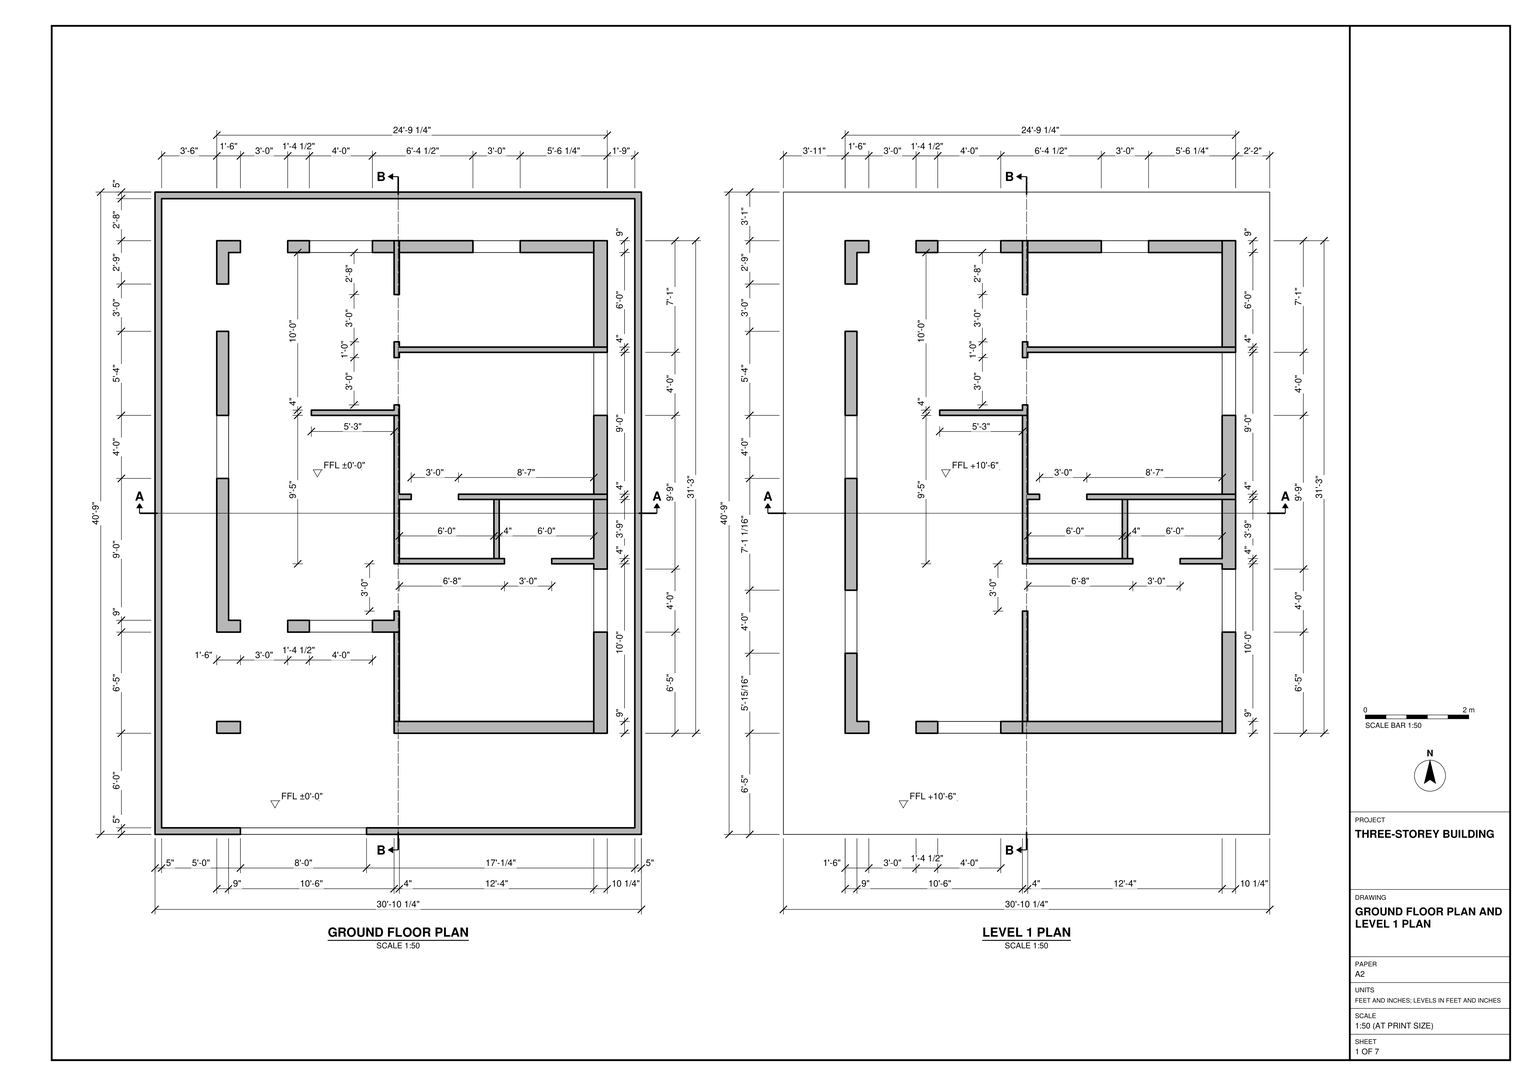
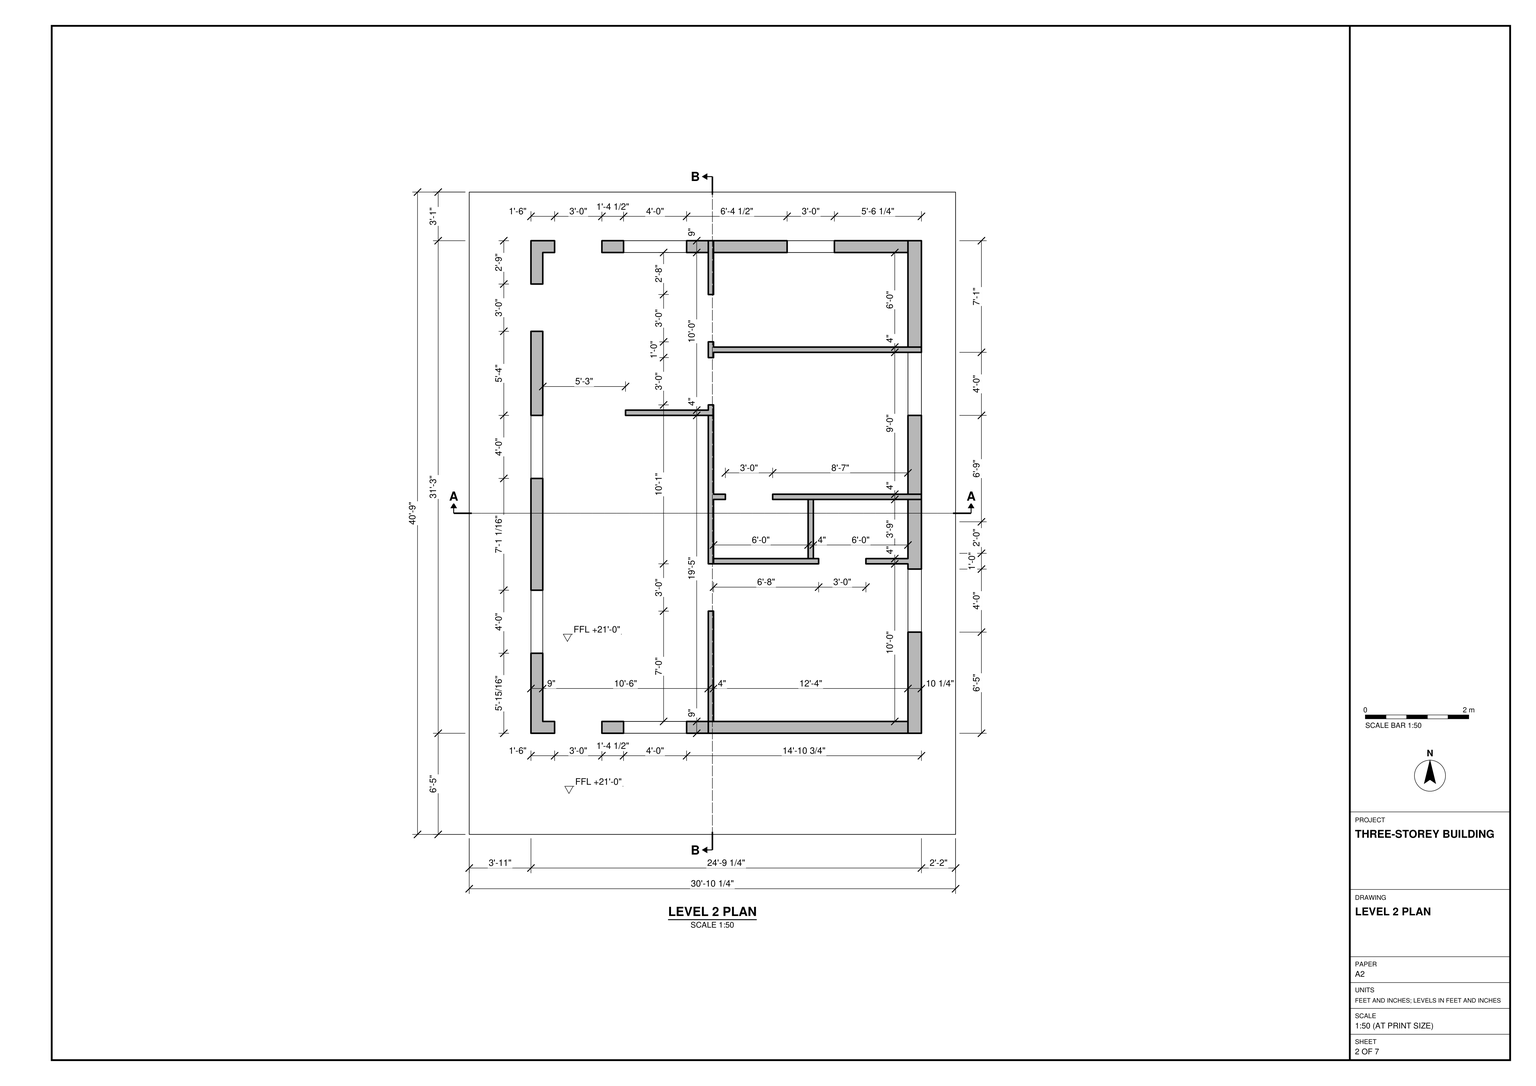
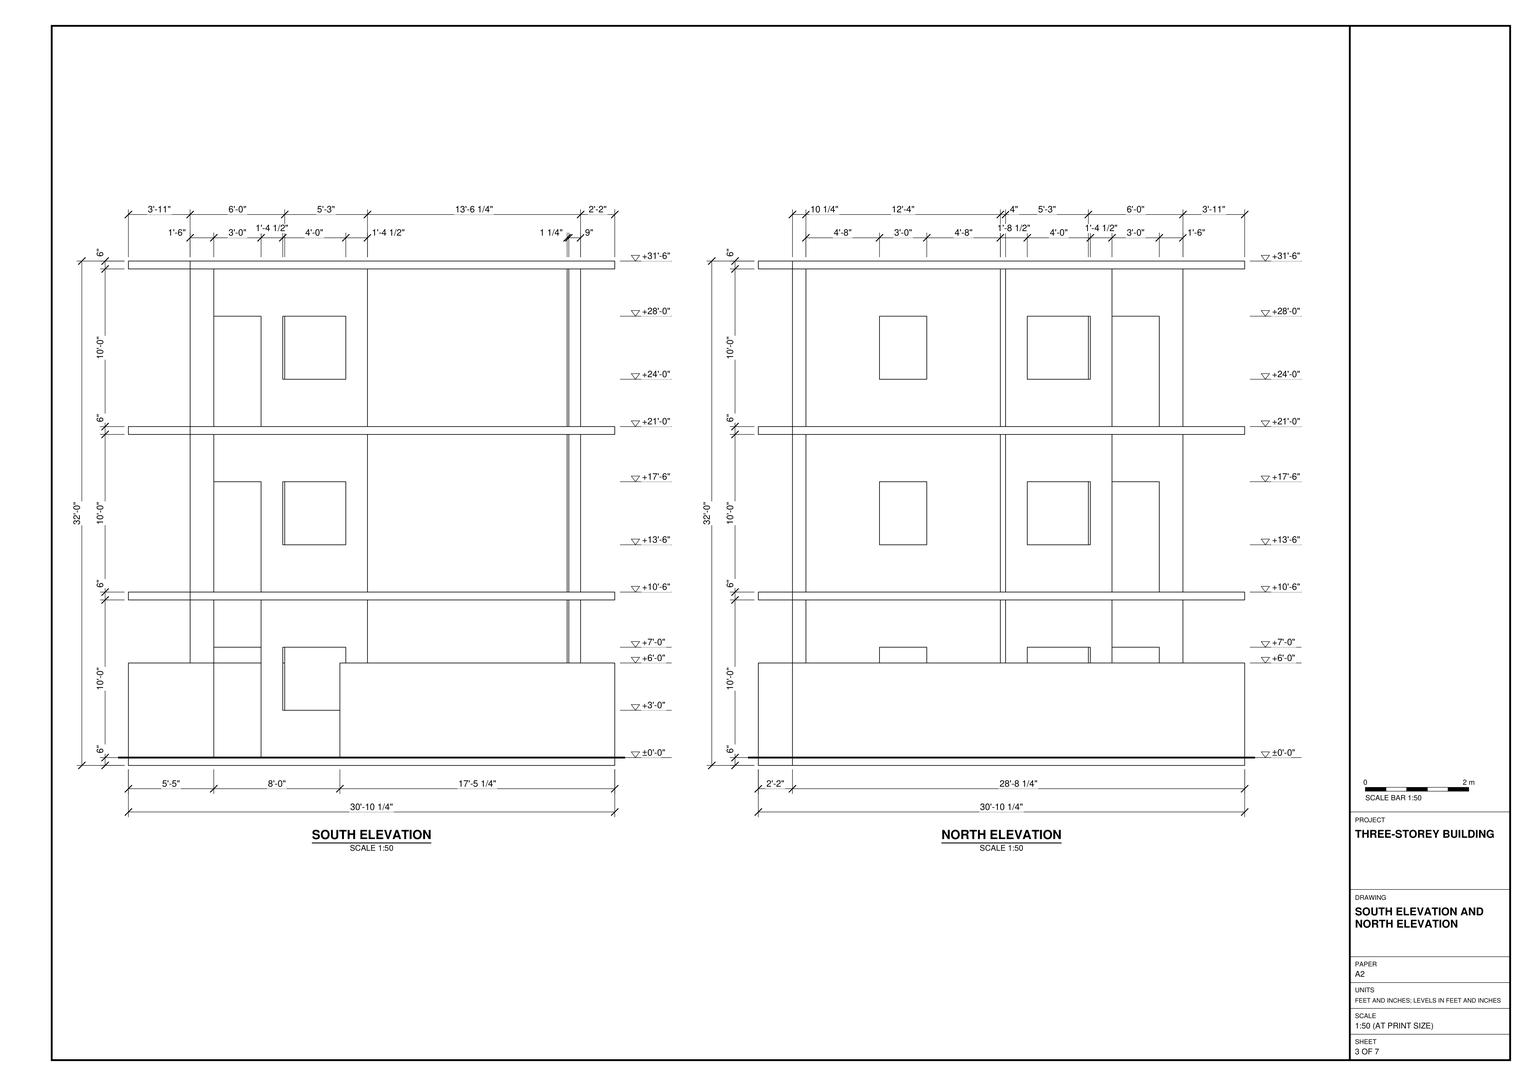
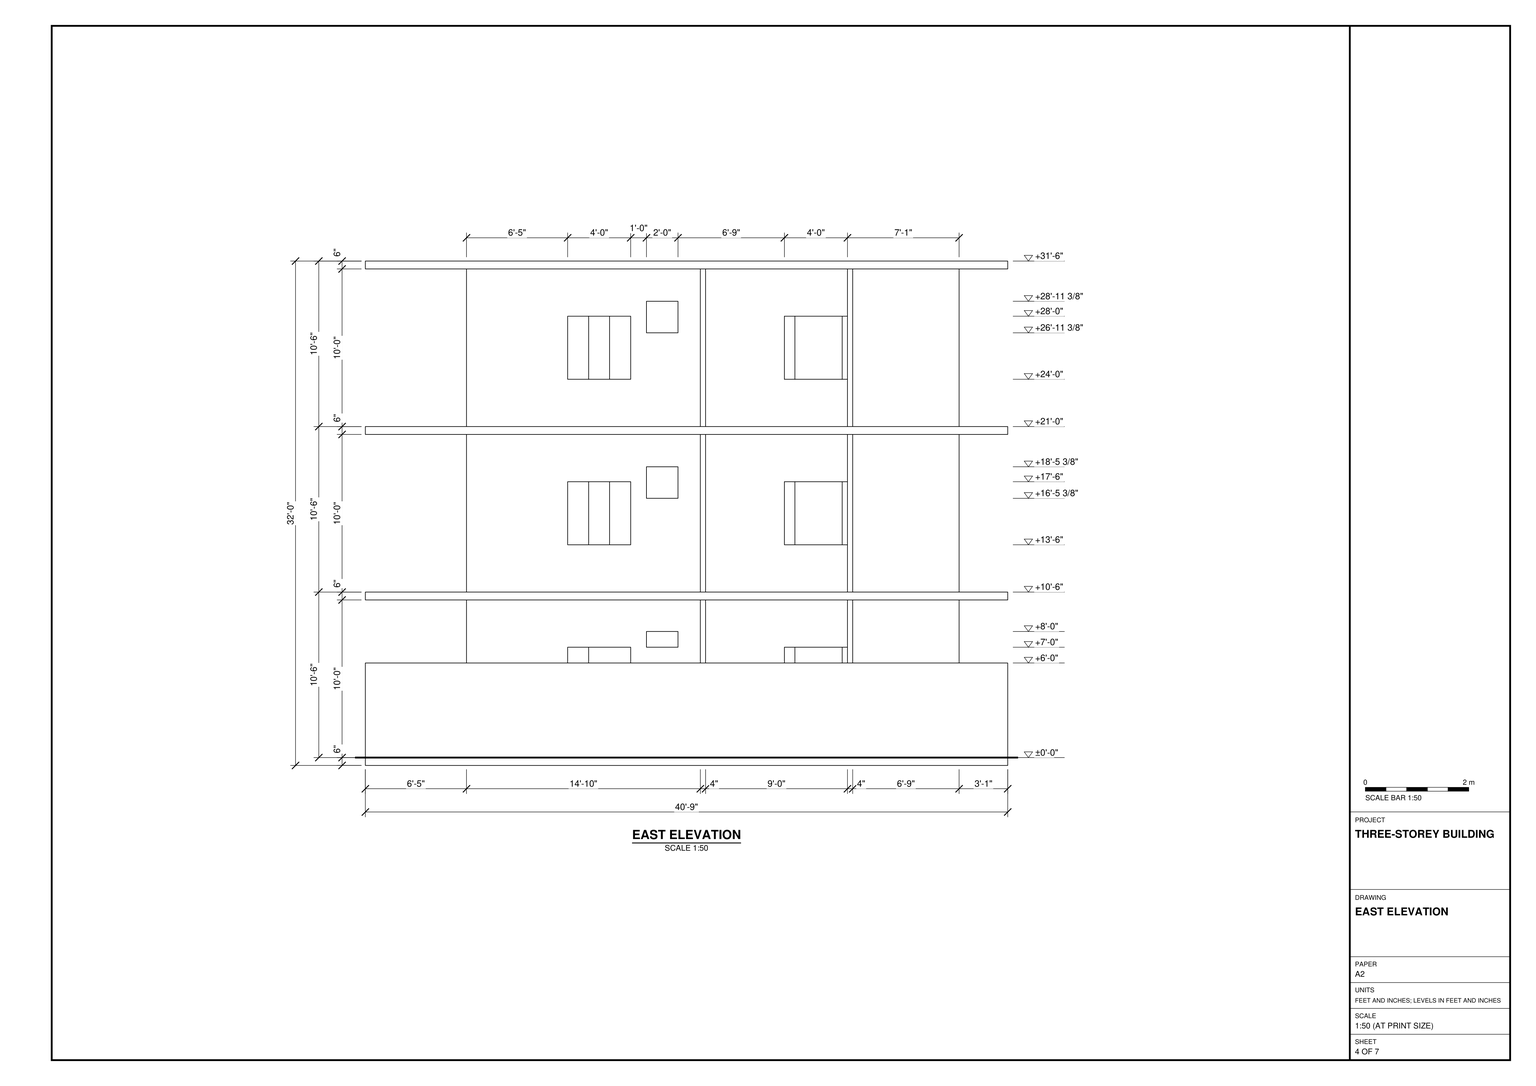
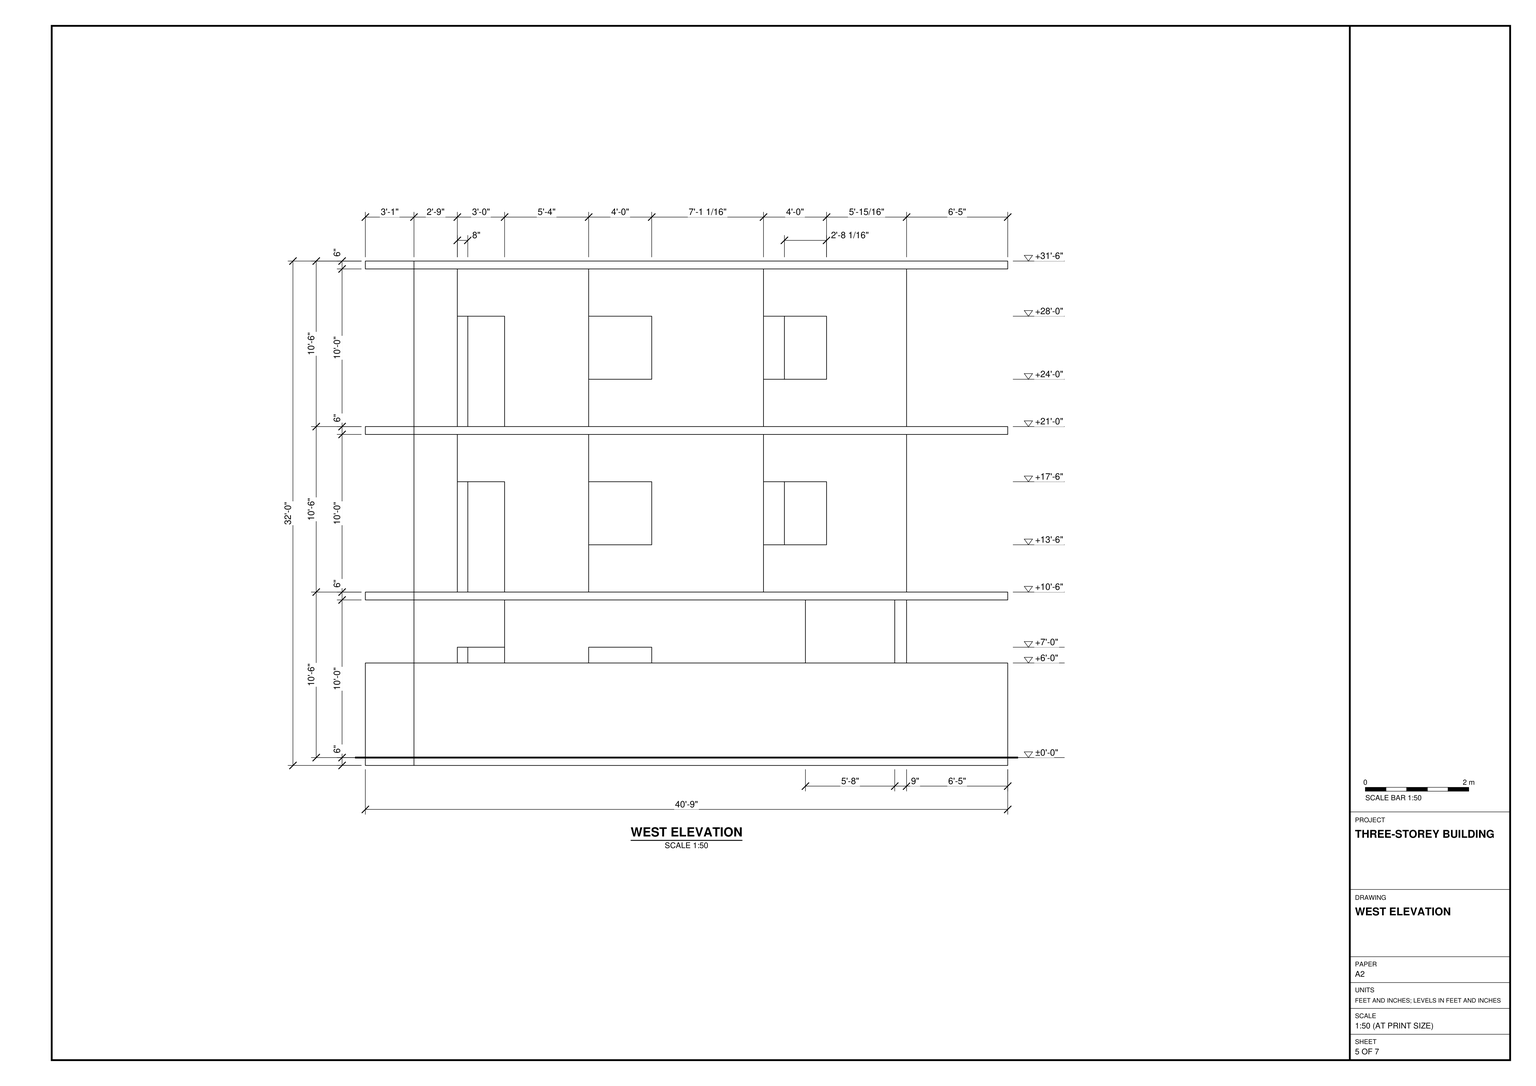
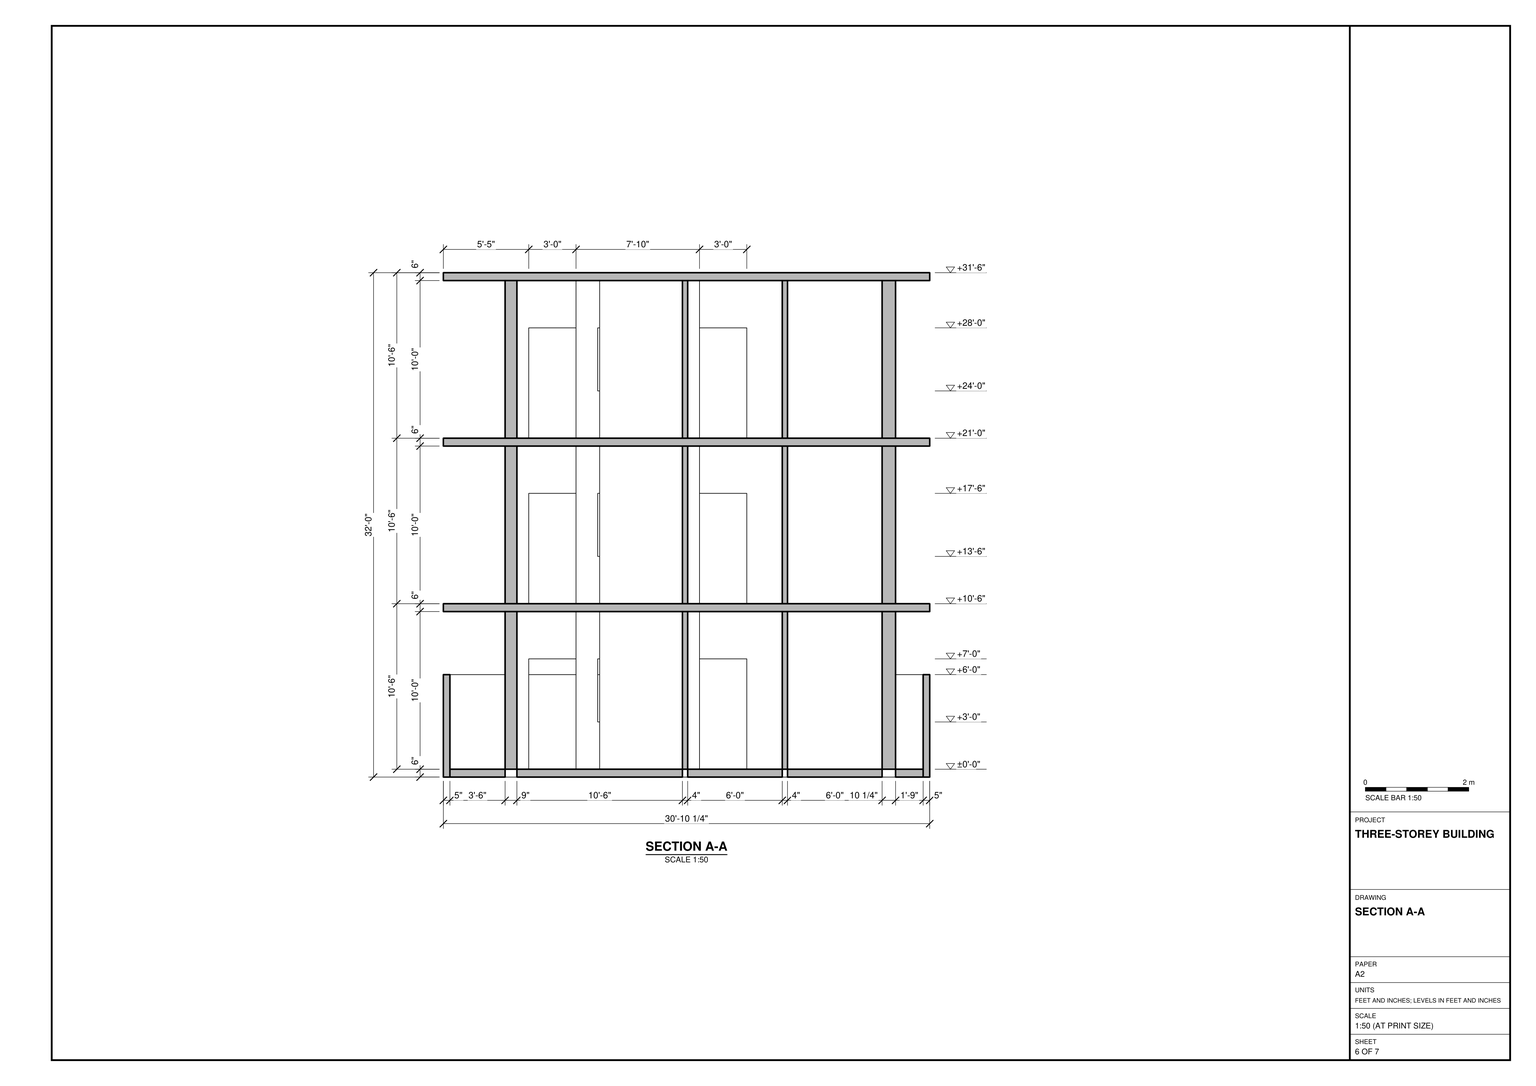
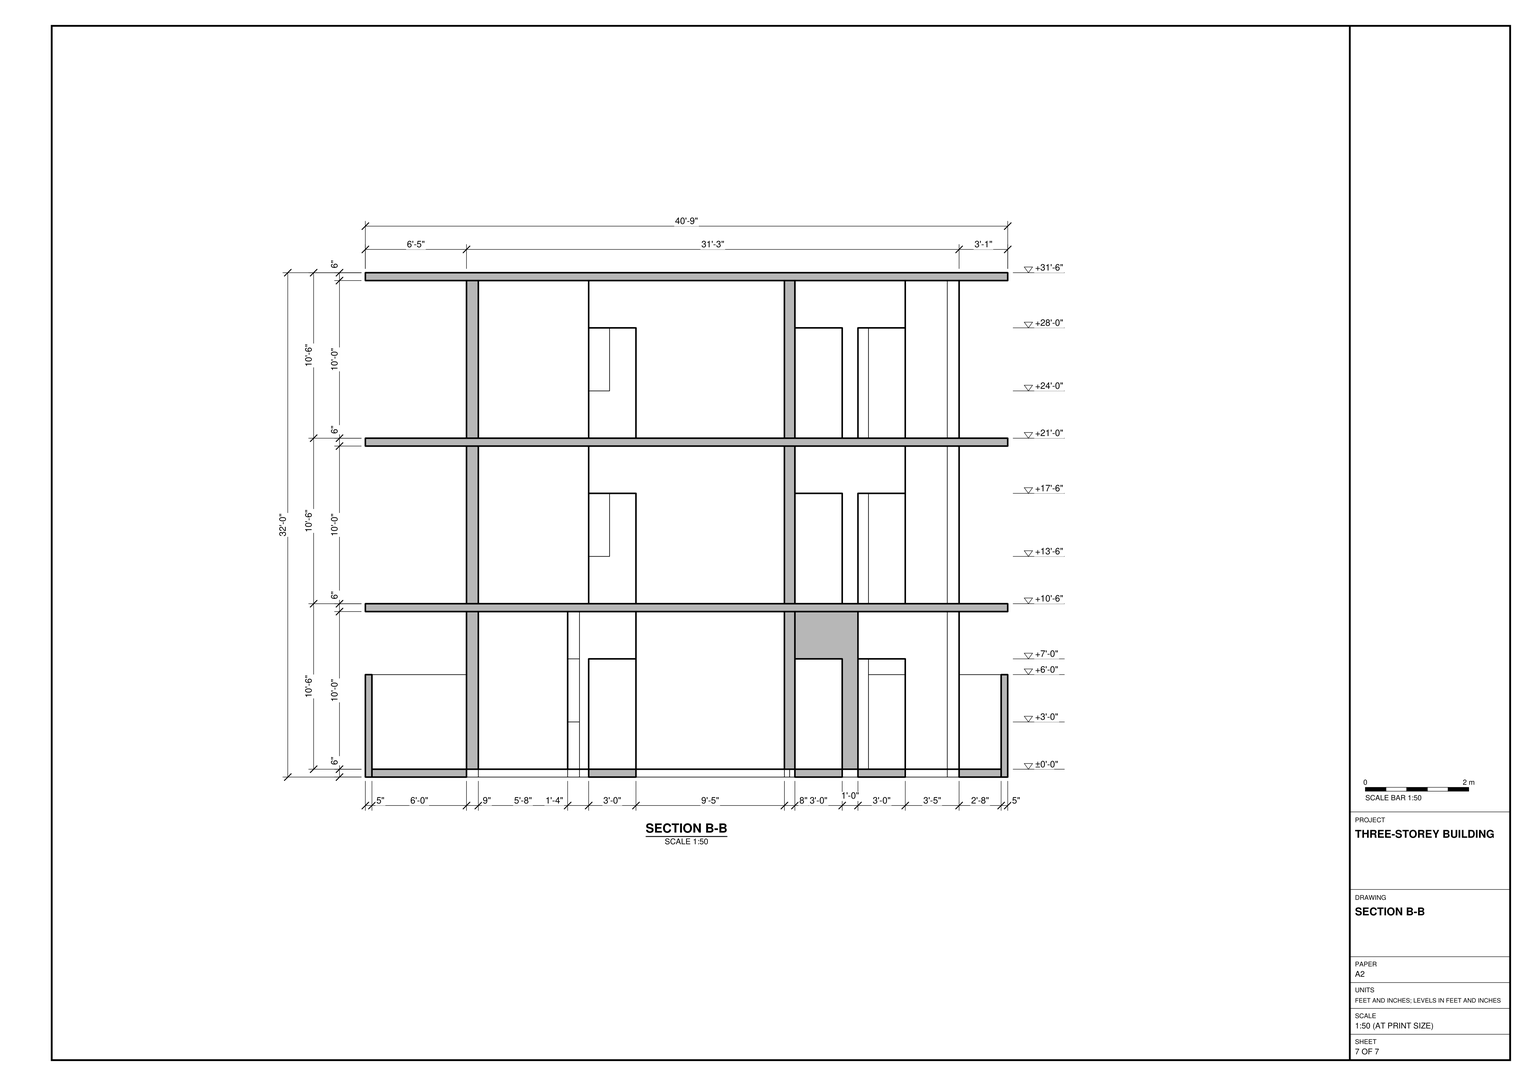
Build the three-storey building in SketchUp from task_files/diagram_01.pdf. Work in feet and inches. The overall model is 30'-10 1/4" wide, 40'-9" deep and 32'-0" high. Set the finished floor levels to ±0'-0", +10'-6" and +21'-0". Measure the overall height from the underside of the ground slab to the top of the flat roof slab.

Lay out the rectangular slabs first. Set the exterior walls back from the slab edges by the different distances shown in plan. At ground level, include the low perimeter wall and its offset entrance on the south side. Reproduce the recessed southwest portion of the ground-floor enclosure and the different wall line above it. Use the drawn thicknesses for the exterior walls and interior partitions. Follow each plan for the room divisions and connecting openings, particularly the pair of small spaces on the east side. Use the elevations to distinguish door openings that reach the floor from windows with raised sills.

Keep walls, slabs, the roof and any furniture or joinery pieces in separate groups or components, and use components for repeated parts. Any decor or loose items shown may be represented by suitable library components. Save one SketchUp model as output_files/three_storey_building_with_projecting_slabs.skp.

# SketchUp Ruby script. Lengths in inches.
U = 1.inch
M = Sketchup.active_model
def pt(a) = Geom::Point3d.new(a.map { |v| v * U })
def face(e, loops, mat)
  f = e.add_face(loops[0].map { |a| pt(a) })
  loops[1..].each { |l| e.add_face(l.map { |a| pt(a) }).erase! }
  f.material = f.back_material = mat if mat
  f
end
# faces: each face lists its corners as indices into pts; further lists are holes
def faces(e, pts, list, mat = nil) = list.each { |f| face(e, (f[0].is_a?(Array) ? f : [f]).map { |l| l.map { |i| pts[i] } }, mat) }
# xy, xz, yz: faces in a plane at the given z, y or x. An outline is a flat list of corners, or four numbers for a rectangle; further outlines are holes
def ring(l) = l.size == 4 ? [[l[0], l[1]], [l[2], l[1]], [l[2], l[3]], [l[0], l[3]]] : l.each_slice(2).to_a
def flat(e, list, mat, &to3) = list.each { |f| face(e, (f[0].is_a?(Array) ? f : [f]).map { |l| ring(l).map { |u, v| to3.(u, v) } }, mat) }
def xy(e, z, list, mat = nil) = flat(e, list, mat) { |x, y| [x, y, z] }
def xz(e, y, list, mat = nil) = flat(e, list, mat) { |x, z| [x, y, z] }
def yz(e, x, list, mat = nil) = flat(e, list, mat) { |y, z| [x, y, z] }
def lines(e, pts, list) = list.each { |a, b| e.add_line(pt(pts[a]), pt(pts[b])) }
# prism: a flat outline (further loops are holes) pulled along v
def prism(e, loops, v, mat = nil)
  f = face(e, loops, mat); d = Geom::Vector3d.new(v.map { |x| x * U })
  f.pushpull(f.normal.samedirection?(d) ? d.length : -d.length)
end
def box(e, o, s, mat = nil) = prism(e, [[o, [o[0] + s[0], o[1], o[2]], [o[0] + s[0], o[1] + s[1], o[2]], [o[0], o[1] + s[1], o[2]]]], [0, 0, s[2]], mat)
def at(x, y, z, deg = 0) = Geom::Transformation.translation(pt([x, y, z])) * Geom::Transformation.rotation(ORIGIN, Z_AXIS, deg.degrees)
def axes(o, x, y, z) = Geom::Transformation.new([*x, 0, *y, 0, *z, 0, *pt(o).to_a, 1])
def part(name) = M.definitions.add(name)
# library, detail: a bought-in or finely detailed component or shape, given as its bounding box
def library(name, o, s) = part(name).tap { |d| box(d.entities, o, s) }
def detail(e, o, s) = box(e.add_group.entities, o, s)
def put(e, d, t, mat = nil) = e.add_instance(d, t).tap { |i| i.material = mat if mat }
def group(e, t, mat = nil) = e.add_group.tap { |g| g.transformation = t; g.material = mat if mat }.entities
root = M.entities
c1 = part("Group\#20")
box(c1.entities,[0,0,0],[4,84,120])
c2 = part("Group\#18")
xy(c2.entities,0,[[0,0,0,108.91,9,108.91,9,9,18,9,18,0],[0,108.91,9,242],[0,242,9,306]])
xy(c2.entities,36,[[0,60.91,9,108.91],[0,194,9,242]])
xy(c2.entities,84,[[0,60.91,9,108.91],[0,194,9,242],[0,306,9,342]])
xy(c2.entities,120,[[0,0,18,0,18,9,9,9,9,342,0,342]])
xz(c2.entities,0,[[0,0,18,120]])
xz(c2.entities,9,[[9,0,18,120]])
xz(c2.entities,60.91,[[0,36,9,84]])
xz(c2.entities,108.91,[[0,36,9,84]])
xz(c2.entities,194,[[0,36,9,84]])
xz(c2.entities,242,[[0,36,9,84]])
xz(c2.entities,306,[[0,0,9,84]])
xz(c2.entities,342,[[0,84,9,120]])
yz(c2.entities,0,[[0,0,0,120,108.91,120,108.91,84,60.91,84,60.91,36,108.91,36,108.91,0],[108.91,0,108.91,120,242,120,242,84,194,84,194,36,242,36,242,0],[242,0,242,120,342,120,342,84,306,84,306,0]])
yz(c2.entities,9,[[[9,0,306,0,306,84,342,84,342,120,9,120],[194,36,242,84],[60.91,36,108.91,84]]])
yz(c2.entities,18,[[0,0,9,120]])
c3 = part("Group\#19")
prism(c3.entities,[[[81,0,0],[81,0,120],[-36,0,120],[-36,0,84],[0,0,84],[0,0,0],[64.5,0,0]],[[16.5,0,84],[64.5,0,84],[64.5,0,36],[16.5,0,36]]],[0,9,0])
c4 = part("Group\#29")
xy(c4.entities,0,[[32,0,42.25,125],[32,125,32,129,0,129,0,133,32,133,32,137,42.25,137,42.25,125],[32,137,42.25,178]])
xy(c4.entities,36,[[32,77,42.25,125]])
xy(c4.entities,71.38,[[32,137,42.25,161]])
xy(c4.entities,84,[[32,77,42.25,125]])
xy(c4.entities,95.38,[[32,137,42.25,161]])
xy(c4.entities,120,[[32,0,42.25,0,42.25,178,32,178,32,133,0,133,0,129,32,129]])
xz(c4.entities,0,[[32,0,33.25,120],[33.25,0,42.25,120]])
xz(c4.entities,77,[[32,36,42.25,84]])
xz(c4.entities,125,[[32,36,42.25,84]])
xz(c4.entities,129,[[0,0,32,120]])
xz(c4.entities,133,[[0,0,32,120]])
xz(c4.entities,137,[[32,71.38,42.25,95.38]])
xz(c4.entities,161,[[32,71.38,42.25,95.38]])
xz(c4.entities,178,[[32,0,42.25,120]])
yz(c4.entities,0,[[129,0,133,120]])
yz(c4.entities,32,[[0,0,9,120],[[9,0,129,120],[77,36,125,84]],[[133,0,178,120],[137,71.38,161,95.38]]])
yz(c4.entities,42.25,[[[0,0,178,120],[77,36,125,84],[137,71.38,161,95.38]]])
p = [[32,167.37,71.85],[42.25,167.37,71.85]]
lines(c4.entities,p,[[0,1]])
c5 = part("Group\#32")
xy(c5.entities,0,[[0,0,0,113,4,113,4,53,13,53,13,49,4,49,4,0]])
xy(c5.entities,84,[[0,-36,4,0]])
xy(c5.entities,120,[[0,-36,4,-36,4,49,13,49,13,53,4,53,4,113,0,113]])
xz(c5.entities,-36,[[0,84,4,120]])
xz(c5.entities,0,[[0,0,4,84]])
xz(c5.entities,49,[[4,0,13,120]])
xz(c5.entities,53,[[4,0,13,120]])
xz(c5.entities,113,[[0,0,4,120]])
yz(c5.entities,0,[[0,0,0,84,-36,84,-36,120,113,120,113,0]])
yz(c5.entities,4,[[0,0,49,0,49,120,-36,120,-36,84,0,84],[53,0,113,120]])
yz(c5.entities,13,[[49,0,53,120]])
c6 = part("Group\#26")
xy(c6.entities,0,[[0,0,0,12,4,12,4,8,162.25,8,162.25,4,4,4,4,0]])
xy(c6.entities,84,[[0,-36,4,0],[0,12,4,48]])
xy(c6.entities,120,[[0,-36,4,-36,4,4,162.25,4,162.25,8,4,8,4,48,0,48]])
xz(c6.entities,-36,[[0,84,4,120]])
xz(c6.entities,0,[[0,0,4,84]])
xz(c6.entities,4,[[4,0,152,120],[152,0,162.25,120]])
xz(c6.entities,8,[[4,0,152,120],[152,0,162.25,120]])
xz(c6.entities,12,[[0,0,4,84]])
xz(c6.entities,48,[[0,84,4,120]])
yz(c6.entities,0,[[0,0,0,84,-36,84,-36,120,48,120,48,84,12,84,12,0]])
yz(c6.entities,4,[[0,0,4,0,4,120,-36,120,-36,84,0,84],[8,0,12,0,12,84,48,84,48,120,8,120]])
yz(c6.entities,162.25,[[4,0,8,120]])
c7 = part("Group\#34")
prism(c7.entities,[[[152,0,0],[0,0,0],[0,9,0],[4,9,0],[152,9,0]]],[0,0,120])
c8 = part("Group\#30")
box(c8.entities,[0,0,0],[4,45,120])
c9 = part("Group\#23")
prism(c9.entities,[[[148,9,0],[92,9,0],[0,9,0],[0,9,120],[148,9,120]],[[56,9,36],[92,9,36],[92,9,84],[56,9,84]]],[0,-9,0])
c10 = part("Group\#21")
xy(c10.entities,0,[[0,0,0,33,18,33,18,24,9,24,9,0]])
xy(c10.entities,84,[[18,24,54,33]])
xy(c10.entities,120,[[0,0,9,0,9,24,54,24,54,33,0,33]])
xz(c10.entities,0,[[0,0,9,120]])
xz(c10.entities,24,[[9,0,18,0,18,84,54,84,54,120,9,120]])
xz(c10.entities,33,[[0,0,0,120,54,120,54,84,18,84,18,0]])
yz(c10.entities,0,[[0,0,33,120]])
yz(c10.entities,9,[[0,0,24,120]])
yz(c10.entities,18,[[24,0,33,84]])
yz(c10.entities,54,[[24,84,33,120]])
c11 = part("Group\#25")
prism(c11.entities,[[[0,81,0],[10.25,81,0],[10.25,0,0],[0,0,0],[0,72,0]]],[0,0,120])
c12 = part("Group\#33")
prism(c12.entities,[[[63,4,0],[63,8,0],[67,8,0],[67,0,0],[0,0,0],[0,4,0]]],[0,0,120])
c13 = part("Group\#22")
prism(c13.entities,[[[81,9,0],[64.5,9,0],[0,9,0],[0,9,120],[81,9,120]],[[16.5,9,36],[64.5,9,36],[64.5,9,84],[16.5,9,84]]],[0,-9,0])
c14 = part("Group\#24")
prism(c14.entities,[[[0,0,0],[0,32,0],[0,41,0],[4,41,0],[4,0,0]]],[0,0,120])
c15 = part("Group\#31")
xy(c15.entities,0,[[0,0,80,4]])
xy(c15.entities,84,[[80,0,116,4]])
xy(c15.entities,120,[[0,0,116,4]])
xz(c15.entities,0,[[0,0,80,0,80,84,116,84,116,120,0,120]])
xz(c15.entities,4,[[0,0,72,120],[72,0,76,120],[76,0,76,120,116,120,116,84,80,84,80,0]])
yz(c15.entities,0,[[0,0,4,120]])
yz(c15.entities,80,[[0,0,4,84]])
yz(c15.entities,116,[[0,84,4,120]])
c16 = part("Group\#28")
xy(c16.entities,0,[[0,0,113.25,4]])
xy(c16.entities,84,[[-36,0,0,4]])
xy(c16.entities,120,[[-36,0,113.25,4]])
xz(c16.entities,0,[[0,0,113.25,0,113.25,120,-36,120,-36,84,0,84]])
xz(c16.entities,4,[[0,0,0,84,-36,84,-36,120,103,120,103,0],[103,0,113.25,120]])
yz(c16.entities,-36,[[0,84,4,120]])
yz(c16.entities,0,[[0,0,4,84]])
yz(c16.entities,113.25,[[0,0,4,120]])
c17 = part("Group\#27")
prism(c17.entities,[[[10.25,0,0],[10.25,108,0],[10.25,108,36],[10.25,60,36],[10.25,60,84],[10.25,108,84],[10.25,108,120],[10.25,0,120]]],[-10.25,0,0])
c18 = part("Group\#36")
prism(c18.entities,[[[0,0,-6],[0,452,-6],[0,489,-6],[344.25,489,-6],[370.25,489,-6],[370.25,0,-6],[47,0,-6]]],[0,0,6])
g1 = group(root,at(47,419,0))
xy(g1,0,[[0,0,0,33,18,33,18,24,9,24,9,0]])
xy(g1,84,[[0,-36,9,0],[18,24,54,33]])
xy(g1,120,[[0,-36,9,-36,9,24,54,24,54,33,0,33]])
xz(g1,-36,[[0,84,9,120]])
xz(g1,0,[[0,0,9,84]])
xz(g1,24,[[9,0,18,0,18,84,54,84,54,120,9,120]])
xz(g1,33,[[0,0,0,120,54,120,54,84,18,84,18,0]])
yz(g1,0,[[0,0,0,84,-36,84,-36,120,33,120,33,0]])
yz(g1,9,[[0,0,24,0,24,120,-36,120,-36,84,0,84]])
yz(g1,18,[[24,0,33,84]])
yz(g1,54,[[24,84,33,120]])
g2 = group(root,at(101,443,0))
prism(g2,[[[0,9,120],[81,9,120],[81,9,0],[64.5,9,0],[0,9,0]],[[64.5,9,36],[64.5,9,84],[16.5,9,84],[16.5,9,36]]],[0,-9,0])
g3 = group(root,at(182,411,0))
xy(g3,0,[[0,0,4,41]])
xy(g3,84,[[0,-36,4,0]])
xy(g3,120,[[0,-36,4,41]])
xz(g3,-36,[[0,84,4,120]])
xz(g3,0,[[0,0,4,84]])
xz(g3,41,[[0,0,4,120]])
yz(g3,0,[[0,0,0,84,-36,84,-36,120,32,120,32,0],[32,0,41,120]])
yz(g3,4,[[0,0,32,0,32,120,-36,120,-36,84,0,84],[32,0,41,120]])
g4 = group(root,at(186,443,0))
prism(g4,[[[148,9,0],[92,9,0],[0,9,0],[0,9,120],[148,9,120]],[[56,9,36],[92,9,36],[92,9,84],[56,9,84]]],[0,-9,0])
g5 = group(root,at(334,371,0))
prism(g5,[[[0,81,0],[10.25,81,0],[10.25,0,0],[0,0,0],[0,72,0]]],[0,0,120])
g6 = group(root,at(182,363,0))
xy(g6,0,[[0,0,0,12,4,12,4,8,162.25,8,162.25,4,4,4,4,0]])
xy(g6,84,[[0,-36,4,0]])
xy(g6,120,[[0,-36,4,-36,4,4,162.25,4,162.25,8,4,8,4,12,0,12]])
xz(g6,-36,[[0,84,4,120]])
xz(g6,0,[[0,0,4,84]])
xz(g6,4,[[4,0,162.25,120]])
xz(g6,8,[[4,0,152,120],[152,0,162.25,120]])
xz(g6,12,[[0,0,4,120]])
yz(g6,0,[[0,0,0,84,-36,84,-36,120,12,120,12,0]])
yz(g6,4,[[0,0,4,0,4,120,-36,120,-36,84,0,84],[8,0,12,120]])
yz(g6,162.25,[[4,0,8,120]])
g7 = group(root,at(334,259,0))
prism(g7,[[[10.25,0,0],[10.25,108,0],[10.25,108,36],[10.25,60,36],[10.25,60,84],[10.25,108,84],[10.25,108,120],[10.25,0,120]]],[-10.25,0,0])
g8 = group(root,at(231,255,0))
xy(g8,0,[[0,0,113.25,4]])
xy(g8,84,[[-36,0,0,4]])
xy(g8,120,[[-36,0,113.25,4]])
xz(g8,0,[[0,0,113.25,0,113.25,120,-36,120,-36,84,0,84]])
xz(g8,4,[[0,0,0,84,-36,84,-36,120,103,120,103,0],[103,0,113.25,120]])
yz(g8,-36,[[0,84,4,120]])
yz(g8,0,[[0,0,4,84]])
yz(g8,113.25,[[0,0,4,120]])
g9 = group(root,at(119,319,0))
prism(g9,[[[63,4,0],[63,8,0],[67,8,0],[67,0,0],[63,0,0],[0,0,0],[0,4,0]]],[0,0,120])
g10 = group(root,at(182,206,0))
prism(g10,[[[4,53,0],[13,53,0],[13,49,0],[4,49,0],[4,4,0],[4,0,0],[0,0,0],[0,113,0],[4,113,0]]],[0,0,120])
g11 = group(root,at(186,206,0))
prism(g11,[[[76,4,0],[80,4,0],[80,0,0],[0,0,0],[0,4,0],[72,4,0]]],[0,0,120])
g12 = group(root,at(258,210,0))
box(g12,[0,0,0],[4,45,120])
g13 = group(root,at(302,77,0))
xy(g13,0,[[32,0,42.25,77],[32,77,32,129,0,129,0,133,32,133,32,161,42.25,161,42.25,77],[32,161,42.25,178]])
xy(g13,36,[[32,77,42.25,125]])
xy(g13,84,[[32,77,42.25,125],[-36,129,0,133],[32,137,42.25,161]])
xy(g13,96,[[32,137,42.25,161]])
xy(g13,120,[[32,0,42.25,0,42.25,178,32,178,32,133,-36,133,-36,129,32,129]])
xz(g13,0,[[32,0,33.25,120],[33.25,0,42.25,120]])
xz(g13,77,[[32,36,42.25,84]])
xz(g13,125,[[32,36,42.25,84]])
xz(g13,129,[[0,0,32,0,32,120,-36,120,-36,84,0,84]])
xz(g13,133,[[0,0,0,84,-36,84,-36,120,32,120,32,0]])
xz(g13,137,[[32,84,42.25,96]])
xz(g13,161,[[32,84,42.25,96]])
xz(g13,178,[[32,0,42.25,120]])
yz(g13,-36,[[129,84,133,120]])
yz(g13,0,[[129,0,133,84]])
yz(g13,32,[[[0,0,129,120],[77,36,125,84]],[[133,0,178,120],[137,84,161,96]]])
yz(g13,42.25,[[[0,0,178,120],[77,36,125,84],[137,84,161,96]]])
g14 = group(root,at(182,77,0))
prism(g14,[[[152,0,0],[0,0,0],[0,9,0],[4,9,0],[152,9,0]]],[0,0,120])
g15 = group(root,at(182,86,0))
box(g15,[0,0,0],[4,68,120])
g16 = group(root,at(101,154,0))
xy(g16,0,[[0,0,16.5,9],[16.5,0,16.5,9,81,9,81,16,85,16,85,0]])
xy(g16,36,[[16.5,0,64.5,9]])
xy(g16,84,[[16.5,0,64.5,9],[81,16,85,52]])
xy(g16,120,[[0,0,85,0,85,52,81,52,81,9,0,9]])
xz(g16,0,[[[0,0,81,120],[16.5,36,64.5,84]],[81,0,85,120]])
xz(g16,9,[[[0,0,81,120],[16.5,36,64.5,84]]])
xz(g16,16,[[81,0,85,84]])
xz(g16,52,[[81,84,85,120]])
yz(g16,0,[[0,0,9,120]])
yz(g16,16.5,[[0,36,9,84]])
yz(g16,64.5,[[0,36,9,84]])
yz(g16,81,[[9,0,9,120,52,120,52,84,16,84,16,0]])
yz(g16,85,[[0,0,16,0,16,84,52,84,52,120,0,120]])
g17 = group(root,at(47,154,0))
xy(g17,0,[[0,0,0,117,9,117,9,9,18,9,18,0],[0,117,9,229]])
xy(g17,36,[[0,117,9,165]])
xy(g17,84,[[18,0,54,9],[0,117,9,165]])
xy(g17,120,[[0,0,54,0,54,9,9,9,9,229,0,229]])
xz(g17,0,[[0,0,18,0,18,84,54,84,54,120,0,120]])
xz(g17,9,[[9,0,9,120,54,120,54,84,18,84,18,0]])
xz(g17,117,[[0,36,9,84]])
xz(g17,165,[[0,36,9,84]])
xz(g17,229,[[0,0,9,120]])
yz(g17,0,[[[0,0,229,120],[117,36,165,84]]])
yz(g17,9,[[[9,0,229,120],[117,36,165,84]]])
yz(g17,18,[[0,0,9,84]])
yz(g17,54,[[0,84,9,120]])
g18 = group(root,at(0,0,113.25))
p = [[117.5,86,12.75],[117.5,77,12.75],[165.5,86,12.75],[165.5,77,12.75],[56,319,12.75],[47,319,12.75],
  [117.5,452,12.75],[117.5,443,12.75],[334,214,12.75],[344.25,214,12.75],[186,367,12.75],[344.25,367,12.75],
  [56,271,12.75],[47,271,12.75],[334,238,12.75],[344.25,238,12.75],[278,443,12.75],[278,452,12.75],
  [242,443,12.75],[242,452,12.75],[334,154,12.75],[344.25,154,12.75],[334,319,12.75],[344.25,319,12.75],
  [334,202,12.75],[344.25,202,12.75],[165.5,452,12.75],[165.5,443,12.75],[56,185.91,12.75],[47,185.91,12.75],
  [56,137.91,12.75],[47,137.91,12.75]]
lines(g18,p,[[0,1],[2,3],[4,5],[6,7],[8,9],[10,11],[12,13],[14,15],[16,17],[18,19],[20,21],[22,23],
  [24,25],[26,27],[28,29],[30,31]])
put(g18,c1,at(182,86,12.75))
put(g18,c2,at(47,77,12.75))
put(g18,c3,at(101,77,12.75))
put(g18,c4,at(302,77,12.75))
put(g18,c5,at(182,206,12.75))
put(g18,c6,at(182,363,12.75))
put(g18,c7,at(182,77,12.75))
put(g18,c8,at(258,210,12.75))
put(g18,c9,at(186,443,12.75))
put(g18,c10,at(47,419,12.75))
put(g18,c11,at(334,371,12.75))
put(g18,c12,at(119,319,12.75))
put(g18,c13,at(101,443,12.75))
put(g18,c14,at(182,411,12.75))
put(g18,c15,at(186,206,12.75))
put(g18,c16,at(231,255,12.75))
put(g18,c17,at(334,259,12.75))
put(g18,c18,at(0,0,12.75))
g19 = group(root,at(0,0,239.25))
p = [[117.5,86,12.75],[117.5,77,12.75],[165.5,86,12.75],[165.5,77,12.75],[56,319,12.75],[47,319,12.75],
  [117.5,452,12.75],[117.5,443,12.75],[334,214,12.75],[344.25,214,12.75],[186,367,12.75],[344.25,367,12.75],
  [56,271,12.75],[47,271,12.75],[334,238,12.75],[344.25,238,12.75],[278,443,12.75],[278,452,12.75],
  [242,443,12.75],[242,452,12.75],[334,154,12.75],[344.25,154,12.75],[334,319,12.75],[344.25,319,12.75],
  [334,202,12.75],[344.25,202,12.75],[165.5,452,12.75],[165.5,443,12.75],[56,185.91,12.75],[47,185.91,12.75],
  [56,137.91,12.75],[47,137.91,12.75]]
lines(g19,p,[[0,1],[2,3],[4,5],[6,7],[8,9],[10,11],[12,13],[14,15],[16,17],[18,19],[20,21],[22,23],
  [24,25],[26,27],[28,29],[30,31]])
put(g19,c1,at(182,86,12.75))
put(g19,c2,at(47,77,12.75))
put(g19,c3,at(101,77,12.75))
put(g19,c4,at(302,77,12.75))
put(g19,c5,at(182,206,12.75))
put(g19,c6,at(182,363,12.75))
put(g19,c7,at(182,77,12.75))
put(g19,c8,at(258,210,12.75))
put(g19,c9,at(186,443,12.75))
put(g19,c10,at(47,419,12.75))
put(g19,c11,at(334,371,12.75))
put(g19,c12,at(119,319,12.75))
put(g19,c13,at(101,443,12.75))
put(g19,c14,at(182,411,12.75))
put(g19,c15,at(186,206,12.75))
put(g19,c16,at(231,255,12.75))
put(g19,c17,at(334,259,12.75))
put(g19,c18,at(0,0,12.75))
put(g19,c18,at(0,0,138.75))
g20 = group(root,at(0,0,0))
box(g20,[47,77,0],[18,9,120])
xy(g20,-6,[[[0,0,370.25,489],[5,5,365.25,484]],[[5,5,365.25,484],[182,77,344.25,77,344.25,452,101,452,101,443,182,443,182,411,186,411,186,443,334,443,334,371,186,371,186,375,182,375,182,363,186,363,186,367,334,367,334,259,231,259,231,255,258,255,258,210,186,210,186,255,195,255,195,259,186,259,186,327,182,327,182,323,119,323,119,319,182,319,182,206,266,206,266,210,262,210,262,255,334,255,334,210,302,210,302,206,334,206,334,86,186,86,186,170,182,170,182,163,101,163,101,154,182,154],[47,154,65,154,65,163,56,163,56,383,47,383]]])
xy(g20,0,[[65,0,161,5],[[5,5,365.25,484],[182,77,182,154,101,154,101,163,182,163,182,170,186,170,186,86,334,86,334,206,302,206,302,210,334,210,334,255,262,255,262,210,266,210,266,206,182,206,182,319,119,319,119,323,182,323,182,327,186,327,186,259,195,259,195,255,186,255,186,210,258,210,258,255,231,255,231,259,334,259,334,367,186,367,186,363,182,363,182,375,186,375,186,371,334,371,334,443,186,443,186,411,182,411,182,443,101,443,101,452,344.25,452,344.25,77],[47,154,47,383,56,383,56,163,65,163,65,154]],[117.5,154,165.5,163],[334,154,344.25,202],[334,214,344.25,238],
  [47,271,56,319],[334,319,344.25,367],[117.5,443,165.5,452],[242,443,278,452]])
xy(g20,72,[[0,0,65,0,65,5,5,5,5,484,365.25,484,365.25,5,161,5,161,0,370.25,0,370.25,489,0,489]])
xz(g20,0,[[0,-6,370.25,-6,370.25,72,161,72,161,0,65,0,65,72,0,72]])
xz(g20,5,[[5,-6,47,0],[47,-6,365.25,0],[5,0,47,72],[47,0,65,72],[161,0,365.25,72]])
xz(g20,77,[[182,-6,334,0],[334,-6,335.25,0],[335.25,-6,344.25,0]])
xz(g20,86,[[186,-6,334,0]])
xz(g20,154,[[47,-6,65,0],[101,-6,117.5,0],[117.5,-6,165.5,0],[165.5,-6,182,0]])
xz(g20,163,[[56,-6,65,0],[101,-6,117.5,0],[117.5,-6,165.5,0],[165.5,-6,182,0]])
xz(g20,170,[[182,-6,186,0]])
xz(g20,206,[[182,-6,186,0],[186,-6,266,0],[302,-6,334,0]])
xz(g20,210,[[186,-6,258,0],[262,-6,266,0],[302,-6,334,0]])
xz(g20,255,[[186,-6,195,0],[231,-6,258,0],[262,-6,334,0]])
xz(g20,259,[[186,-6,195,0],[231,-6,334,0]])
xz(g20,319,[[119,-6,182,0]])
xz(g20,323,[[119,-6,182,0]])
xz(g20,327,[[182,-6,186,0]])
xz(g20,363,[[182,-6,186,0]])
xz(g20,367,[[186,-6,334,0]])
xz(g20,371,[[186,-6,334,0]])
xz(g20,375,[[182,-6,186,0]])
xz(g20,383,[[47,-6,56,0]])
xz(g20,411,[[182,-6,186,0]])
xz(g20,443,[[101,-6,117.5,0],[117.5,-6,165.5,0],[165.5,-6,182,0],[186,-6,242,0],[242,-6,278,0],
  [278,-6,334,0]])
xz(g20,452,[[101,-6,117.5,0],[117.5,-6,165.5,0],[165.5,-6,182,0],[182,-6,186,0],[186,-6,242,0],
  [242,-6,278,0],[278,-6,334,0],[334,-6,344.25,0]])
xz(g20,484,[[5,-6,344.25,0],[344.25,-6,365.25,0],[5,0,344.25,72],[344.25,0,365.25,72]])
xz(g20,489,[[0,-6,344.25,72],[344.25,-6,370.25,72]])
yz(g20,0,[[0,-6,452,72],[452,-6,489,72]])
yz(g20,5,[[5,-6,452,0],[452,-6,484,0],[5,0,452,72],[452,0,484,72]])
yz(g20,47,[[154,-6,271,0],[271,-6,319,0],[319,-6,383,0]])
yz(g20,56,[[163,-6,271,0],[271,-6,319,0],[319,-6,383,0]])
yz(g20,65,[[154,-6,163,0],[0,0,5,72]])
yz(g20,101,[[154,-6,163,0],[443,-6,452,0]])
yz(g20,119,[[319,-6,323,0]])
yz(g20,161,[[0,0,5,72]])
yz(g20,182,[[77,-6,86,0],[86,-6,154,0],[163,-6,170,0],[206,-6,319,0],[323,-6,327,0],
  [363,-6,375,0],[411,-6,443,0]])
yz(g20,186,[[86,-6,154,0],[154,-6,170,0],[210,-6,255,0],[259,-6,319,0],[319,-6,327,0],
  [363,-6,367,0],[371,-6,375,0],[411,-6,443,0]])
yz(g20,195,[[255,-6,259,0]])
yz(g20,231,[[255,-6,259,0]])
yz(g20,258,[[210,-6,255,0]])
yz(g20,262,[[210,-6,255,0]])
yz(g20,266,[[206,-6,210,0]])
yz(g20,302,[[206,-6,210,0]])
yz(g20,334,[[86,-6,154,0],[154,-6,202,0],[202,-6,206,0],[210,-6,214,0],[214,-6,238,0],
  [238,-6,255,0],[259,-6,319,0],[319,-6,367,0],[371,-6,443,0]])
yz(g20,344.25,[[77,-6,154,0],[154,-6,202,0],[202,-6,214,0],[214,-6,238,0],[238,-6,255,0],
  [255,-6,259,0],[259,-6,319,0],[319,-6,367,0],[367,-6,371,0],[371,-6,452,0]])
yz(g20,365.25,[[5,-6,484,0],[5,0,484,72]])
yz(g20,370.25,[[0,-6,489,72]])
